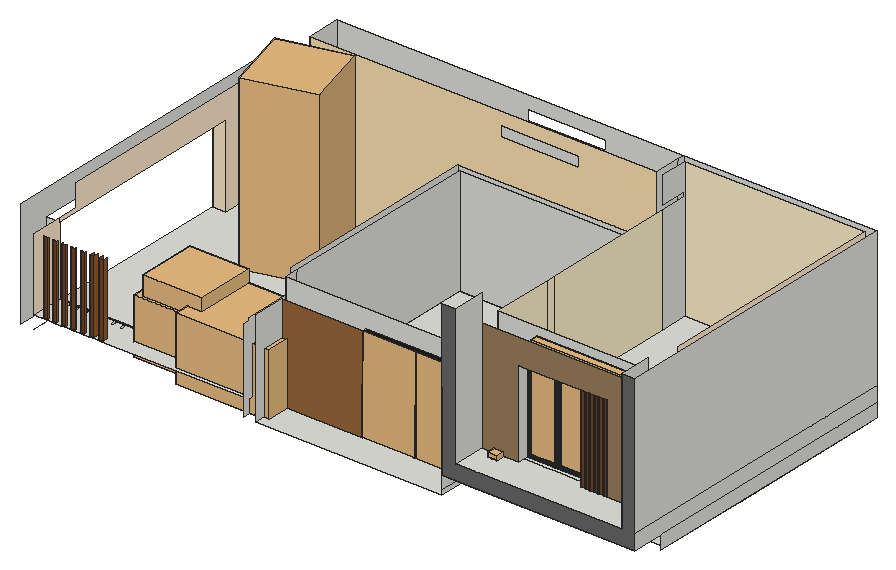
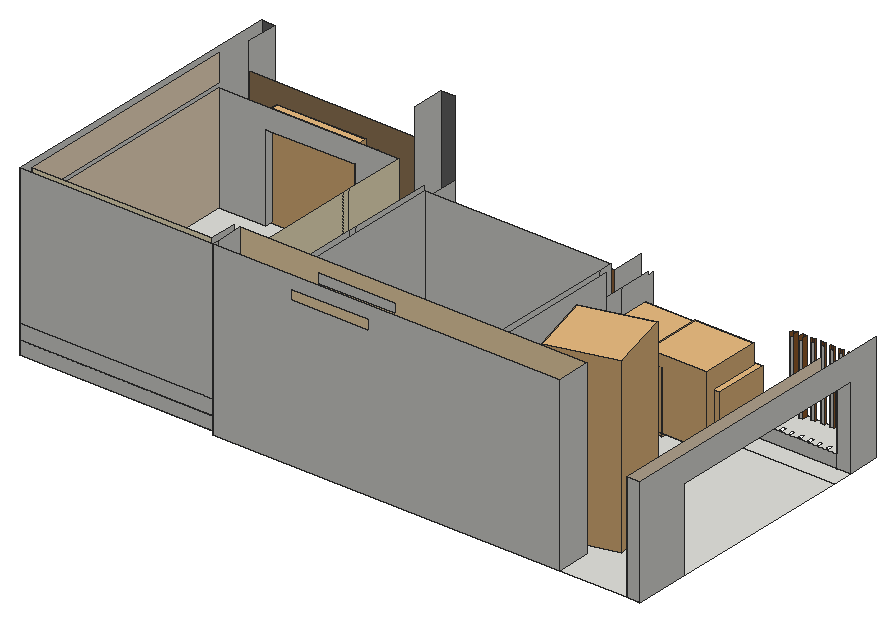
# SketchUp Ruby script. Lengths in inches.
U = 1.inch
M = Sketchup.active_model
def pt(a) = Geom::Point3d.new(a.map { |v| v * U })
def face(e, loops, mat)
  f = e.add_face(loops[0].map { |a| pt(a) })
  loops[1..].each { |l| e.add_face(l.map { |a| pt(a) }).erase! }
  f.material = f.back_material = mat if mat
  f
end
# faces: each face lists its corners as indices into pts; further lists are holes
def faces(e, pts, list, mat = nil) = list.each { |f| face(e, (f[0].is_a?(Array) ? f : [f]).map { |l| l.map { |i| pts[i] } }, mat) }
# xy, xz, yz: faces in a plane at the given z, y or x. An outline is a flat list of corners, or four numbers for a rectangle; further outlines are holes
def ring(l) = l.size == 4 ? [[l[0], l[1]], [l[2], l[1]], [l[2], l[3]], [l[0], l[3]]] : l.each_slice(2).to_a
def flat(e, list, mat, &to3) = list.each { |f| face(e, (f[0].is_a?(Array) ? f : [f]).map { |l| ring(l).map { |u, v| to3.(u, v) } }, mat) }
def xy(e, z, list, mat = nil) = flat(e, list, mat) { |x, y| [x, y, z] }
def xz(e, y, list, mat = nil) = flat(e, list, mat) { |x, z| [x, y, z] }
def yz(e, x, list, mat = nil) = flat(e, list, mat) { |y, z| [x, y, z] }
def lines(e, pts, list) = list.each { |a, b| e.add_line(pt(pts[a]), pt(pts[b])) }
# prism: a flat outline (further loops are holes) pulled along v
def prism(e, loops, v, mat = nil)
  f = face(e, loops, mat); d = Geom::Vector3d.new(v.map { |x| x * U })
  f.pushpull(f.normal.samedirection?(d) ? d.length : -d.length)
end
def box(e, o, s, mat = nil) = prism(e, [[o, [o[0] + s[0], o[1], o[2]], [o[0] + s[0], o[1] + s[1], o[2]], [o[0], o[1] + s[1], o[2]]]], [0, 0, s[2]], mat)
def at(x, y, z, deg = 0) = Geom::Transformation.translation(pt([x, y, z])) * Geom::Transformation.rotation(ORIGIN, Z_AXIS, deg.degrees)
def axes(o, x, y, z) = Geom::Transformation.new([*x, 0, *y, 0, *z, 0, *pt(o).to_a, 1])
def part(name) = M.definitions.add(name)
# library, detail: a bought-in or finely detailed component or shape, given as its bounding box
def library(name, o, s) = part(name).tap { |d| box(d.entities, o, s) }
def detail(e, o, s) = box(e.add_group.entities, o, s)
def put(e, d, t, mat = nil) = e.add_instance(d, t).tap { |i| i.material = mat if mat }
def group(e, t, mat = nil) = e.add_group.tap { |g| g.transformation = t; g.material = mat if mat }.entities
root = M.entities
M.materials.add("Wine2").color = [0, 0, 0]
M.materials["Wine2"].alpha = 0
M.materials.add("[0029_BlanchedAlmond]").color = [255, 235, 205]
M.materials.add("[0032_Moccasin]").color = [255, 228, 181]
M.materials.add("[0130_Gainsboro]").color = [39, 45, 50]
M.materials.add("[0134_DimGray]").color = [105, 105, 105]
M.materials.add("[Color D01]").color = [255, 242, 204]
M.materials.add("[Color M08]").color = [30, 30, 30]
M.materials.add("[Groundcover Sand Smooth]").color = [158, 128, 93]
M.materials.add("[Wood Floor Dark]").color = [153, 94, 42]
M.materials.add("[Wood Floor]").color = [155, 105, 61]
M.materials.add("[Wood Veneer 01]").color = [120, 70, 37]
c1 = library("Sem+nome (1)",[20.77,3.52,-2.22],[96.42,122.82,82.56])
c2 = library("Pot+Plant",[-20.81,-17.08,-0.03],[39.86,39.43,41.33])
c3 = library("staircases+paint",[157.6875,-222.19,0],[58.28,58.28,145.51])
c4 = library("1",[3.97,34.78,0],[101.43,33.99,0.79])
c5 = library("Floor plant",[-5.56,-16.3125,0.81],[76.88,76.71,92.33])
c6 = library("A$C06767DEF\#1",[-8.3,1.21,0],[7.09,7.09,5.51])
c7 = library("oeillet+feston+nino+blanc",[0,-1.53,0],[95.37,7.9,110.56])
c8 = part("Framed panel")
xy(c8.entities,0,[[0,-0.98,43.07,0],[0,0,43.07,1.4]],"[0130_Gainsboro]")
xy(c8.entities,0.3,[[0.3,-1.43,42.77,-0.98]],"[0130_Gainsboro]")
xy(c8.entities,2.95,[[2.95,-1.43,40.12,-0.63],[2.95,-0.63,40.12,0],[2.95,0,40.12,0.64],[2.95,0.64,40.12,1.4]],"[0130_Gainsboro]")
xy(c8.entities,3.54,[[3.54,-0.63,39.53,0],[3.54,0,39.53,0.64]],"[0130_Gainsboro]")
xy(c8.entities,111.8125,[[3.54,-0.63,39.53,0],[3.54,0,39.53,0.64]],"[0130_Gainsboro]")
xy(c8.entities,112.4,[[2.95,-1.43,40.12,-0.63],[2.95,-0.63,40.12,0],[2.95,0,40.12,0.64],[2.95,0.64,40.12,1.4]],"[0130_Gainsboro]")
xy(c8.entities,115.05,[[0.3,-1.43,42.77,-0.98]],"[0130_Gainsboro]")
xy(c8.entities,115.35,[[0,-0.98,43.07,0],[0,0,43.07,1.4]],"[0130_Gainsboro]")
xz(c8.entities,-1.43,[[[0.3,0.3,42.77,115.05],[2.95,2.95,40.12,112.4]]],"[0130_Gainsboro]")
xz(c8.entities,-0.98,[[[0,0,43.07,115.35],[0.3,0.3,42.77,115.05]]],"[0130_Gainsboro]")
xz(c8.entities,-0.63,[[[2.95,2.95,40.12,112.4],[3.54,3.54,39.53,111.8125]]],"[0130_Gainsboro]")
xz(c8.entities,0,[[3.54,3.54,39.53,111.8125]],"Wine2")
xz(c8.entities,0,[[[0,0,43.07,115.35],[2.95,2.95,40.12,112.4]],[[2.95,2.95,40.12,112.4],[3.54,3.54,39.53,111.8125]]],"[0130_Gainsboro]")
xz(c8.entities,0.64,[[[2.95,2.95,40.12,112.4],[3.54,3.54,39.53,111.8125]]],"[0130_Gainsboro]")
xz(c8.entities,1.4,[[[0,0,43.07,115.35],[2.95,2.95,40.12,112.4]]],"[0130_Gainsboro]")
yz(c8.entities,0,[[-0.98,0,0,115.35],[0,0,1.4,115.35]],"[0130_Gainsboro]")
yz(c8.entities,0.3,[[-1.43,0.3,-0.98,115.05]],"[0130_Gainsboro]")
yz(c8.entities,2.95,[[-1.43,2.95,-0.63,112.4],[-0.63,2.95,0,112.4],[0,2.95,0.64,112.4],[0.64,2.95,1.4,112.4]],"[0130_Gainsboro]")
yz(c8.entities,3.54,[[-0.63,3.54,0,111.8125],[0,3.54,0.64,111.8125]],"[0130_Gainsboro]")
yz(c8.entities,39.53,[[-0.63,3.54,0,111.8125],[0,3.54,0.64,111.8125]],"[0130_Gainsboro]")
yz(c8.entities,40.12,[[-1.43,2.95,-0.63,112.4],[-0.63,2.95,0,112.4],[0,2.95,0.64,112.4],[0.64,2.95,1.4,112.4]],"[0130_Gainsboro]")
yz(c8.entities,42.77,[[-1.43,0.3,-0.98,115.05]],"[0130_Gainsboro]")
yz(c8.entities,43.07,[[-0.98,0,0,115.35],[0,0,1.4,115.35]],"[0130_Gainsboro]")
c9 = part("Framed panel assembly")
put(c9.entities,c8,axes([90.57,1.43,0],[1.05148,0,0],[0,1,0],[0,0,1]))
put(c9.entities,c8,axes([0,1.43,0],[1.05148,0,0],[0,1,0],[0,0,1]))
put(c9.entities,c8,axes([45.29,1.43,0],[1.05148,0,0],[0,1,0],[0,0,1]))
xy(root,146.375,[[416.52,389.67,660.05,389.67,660.05,437.41,522.24,437.41,522.24,431.86,416.52,431.86],[522.24,437.41,660.05,440.22],[101.6875,440.22,400.76,466.49],[[400.76,440.22,660.05,739.86],[408.8,448.26,652.01,731.82]],[408.8,448.26,652.01,731.82],
  [101.6875,466.49,400.76,466.49,400.76,739.86,207.07,739.86,207.07,784.05,118.89,784.05,118.89,712.1,101.6875,712.1],[101.6875,712.1,118.89,784.05],[207.07,739.86,660.05,784.05]])
xy(root,151.4375,[[660.05,440.22,666.61,551.1875],[666.61,440.22,904.08,551.1875],[904.08,440.22,912.4375,551.1875],[660.05,551.1875,666.61,562.07],[666.61,551.1875,904.08,562.07],
  [904.08,551.1875,912.4375,562.07],[660.05,562.07,904.08,775.6875],[904.08,562.07,912.4375,775.6875],[660.05,775.6875,912.4375,784.05]])
xy(root,163.5625,[[[118.89,397.92,130.43,397.92,130.43,401.21,135.74,401.21,135.74,397.92,142.61,397.92,142.61,401.21,147.93,401.21,147.93,397.92,154.8,397.92,154.8,401.21,160.11,401.21,160.11,397.92,166.99,397.92,166.99,401.21,172.3,401.21,172.3,397.92,179.18,397.92,179.18,401.21,184.49,401.21,184.49,397.92,191.36,397.92,191.36,405.64,196.68,405.64,196.68,397.92,203.55,397.92,203.55,405.01,208.86,405.01,208.86,397.92,400.76,397.92,400.76,440.22,118.89,440.22],[179.18,431.86,184.49,438.86],[203.55,431.86,208.86,438.86],[191.36,431.86,196.68,438.86],[130.43,431.86,135.74,438.86],[166.99,431.86,172.3,438.86],[142.61,431.86,147.93,438.86],[154.8,431.86,160.11,438.86]],[130.43,397.92,135.74,399.67],[142.61,397.92,147.93,399.67],[154.8,397.92,160.11,399.67],[166.99,397.92,172.3,399.67],
  [179.18,397.92,184.49,399.67],[191.36,397.92,196.68,399.67],[203.55,397.92,208.86,399.67]])
xy(root,169.25,[[660.05,389.67,660.05,784.05,912.4375,784.05,912.4375,431.86,798.1,431.86,798.1,432.24,795.91,432.24,795.91,431.86,720.28,431.86,720.28,432.24,713.72,432.24,713.72,433.11,711.84,433.11,711.84,432.24,705.28,432.24,705.28,433.11,703.41,433.11,703.41,432.17,696.84,432.17,696.84,433.11,694.97,433.11,694.97,432.17,688.41,432.17,688.41,433.11,686.53,433.11,686.53,432.17,679.97,432.17,679.97,433.11,678.11,433.11,678.11,389.67]])
xy(root,169.25,[[678.11,389.67,678.11,433.11,679.97,433.11,679.97,432.17,686.53,432.17,686.53,433.11,688.41,433.11,688.41,432.17,694.97,432.17,694.97,433.11,696.84,433.11,696.84,432.17,703.41,432.17,703.41,433.11,705.28,433.11,705.28,432.24,711.84,432.24,711.84,433.11,713.72,433.11,713.72,432.24,720.28,432.24,720.28,431.86,795.91,431.86,795.91,432.24,798.1,432.24,798.1,431.86,912.4375,431.86,912.4375,389.67]],"[Wood Floor Dark]")
xy(root,185.875,[[699.62,420.82,701.17,421.02,702.625,421.62,703.87,422.56,704.83,423.8,705.43,425.25,705.64,426.8,705.45,428.35,704.85,429.8,703.9,431.05,702.86,431.86,696.44,431.86,695.42,431.08,694.46,429.85,693.86,428.4,693.64,426.85,693.84,425.29,694.4375,423.85,695.39,422.6,696.625,421.64,698.07,421.03],[875.48,421.71,877.03,421.92,878.48,422.52,879.72,423.47,880.67,424.71,881.27,426.16,881.48,427.71,881.27,429.27,880.67,430.71,879.79,431.86,871.16,431.86,870.28,430.71,869.68,429.27,869.48,427.71,869.68,426.16,870.28,424.71,871.23,423.47,872.48,422.52,873.92,421.92]])
xy(root,188.9375,[[[678.11,389.67,895.55,389.67,895.55,431.86,879.79,431.86,880.67,430.71,881.27,429.27,881.48,427.71,881.27,426.16,880.67,424.71,879.72,423.47,878.48,422.52,877.03,421.92,875.48,421.71,873.92,421.92,872.48,422.52,871.23,423.47,870.28,424.71,869.68,426.16,869.48,427.71,869.68,429.27,870.28,430.71,871.16,431.86,837.78,431.86,837.78,434.99,842.22,434.99,842.22,440.41,726.09,440.41,726.09,431.86,702.86,431.86,703.9,431.05,704.85,429.8,705.45,428.35,705.64,426.8,705.43,425.25,704.83,423.8,703.87,422.56,702.625,421.62,701.17,421.02,699.62,420.82,698.07,421.03,696.625,421.64,695.39,422.6,694.4375,423.85,693.84,425.29,693.64,426.85,693.86,428.4,694.46,429.85,695.42,431.08,696.44,431.86,678.11,431.86],[807.9,431.86,812.34,434.99],[813.9,431.86,818.34,434.99],[819.9,431.86,824.34,434.99],[825.9,431.86,830.34,434.99],[831.78,431.86,836.22,434.99]],[696.44,431.86,702.86,431.86,702.67,432.01,701.22,432.61,699.67,432.82,698.12,432.625,696.67,432.03],[871.16,431.86,879.79,431.86,879.72,431.96,878.48,432.91,877.03,433.51,875.48,433.71,873.92,433.51,872.48,432.91,871.23,431.96],[726.09,440.41,842.22,440.41,842.22,469.66,903.88,469.66,903.88,775.49,668.6,775.49,668.6,469.66,726.09,469.66]])
xz(root,389.67,[[660.05,169.25,912.4375,169.25,912.4375,370.4375,895.55,370.4375,895.55,188.9375,678.11,188.9375,678.11,370.4375,660.05,370.4375]],"[0134_DimGray]")
xz(root,399.67,[[130.43,163.5625,135.74,258.66],[142.61,163.5625,147.93,258.66],[154.8,163.5625,160.11,258.66],[166.99,163.5625,172.3,258.66],[179.18,163.5625,184.49,258.66],
  [191.36,163.5625,196.68,258.66],[203.55,163.5625,208.86,258.66]],"[Wood Veneer 01]")
xz(root,401.21,[[130.43,163.5625,135.74,254.91],[142.61,163.5625,147.93,254.91],[154.8,163.5625,160.11,254.91],[166.99,163.5625,172.3,254.91],[179.18,163.5625,184.49,254.91]])
xz(root,405.01,[[203.55,163.5625,208.86,254.91]])
xz(root,405.64,[[191.36,163.5625,196.68,254.91]])
xz(root,431.86,[[696.44,185.875,702.86,188.9375],[871.16,185.875,879.79,188.9375]])
xz(root,431.86,[[678.11,188.9375,726.09,188.9375,726.09,302.375,842.22,302.375,842.22,188.9375,895.55,188.9375,895.55,335.3125,678.11,335.3125]],"[Groundcover Sand Smooth]")
xz(root,431.86,[[416.52,146.375,522.24,271.24]],"[Wood Floor]")
xz(root,431.86,[[807.9,188.9375,812.34,302.375],[813.9,188.9375,818.34,302.375],[819.9,188.9375,824.34,302.375],[825.9,188.9375,830.34,302.375],[831.78,188.9375,836.22,302.375],
  [837.78,188.9375,842.22,302.375]],"[Wood Veneer 01]")
xz(root,434.99,[[807.9,188.9375,812.34,302.375],[813.9,188.9375,818.34,302.375],[819.9,188.9375,824.34,302.375],[825.9,188.9375,830.34,302.375],[831.78,188.9375,836.22,302.375],
  [837.78,188.9375,842.22,302.375]])
xz(root,437.41,[[522.24,146.375,660.05,271.24]],"[Color M08]")
xz(root,440.22,[[101.6875,146.375,118.89,253.6875],[118.89,146.375,400.76,163.5625]])
xz(root,448.26,[[408.8,146.375,652.01,287.5625]])
xz(root,469.66,[[668.6,188.9375,668.6,329.3125,903.88,329.3125,903.88,188.9375,842.22,188.9375,842.22,302.375,726.09,302.375,726.09,188.9375]])
xz(root,712.1,[[101.6875,146.375,118.89,253.6875]],"[0029_BlanchedAlmond]")
xz(root,731.82,[[408.8,146.375,652.01,287.5625]])
xz(root,739.86,[[400.76,146.375,660.05,287.5625]])
xz(root,739.86,[[[207.07,146.375,400.76,146.375,400.76,287.5625,660.05,287.5625,660.05,370.4375,207.07,370.4375],[456.09,340.08,558.27,353.76]]],"[0032_Moccasin]")
xz(root,775.49,[[668.6,188.9375,903.88,370.4375]],"[Color D01]")
xz(root,784.05,[[101.6875,146.375,118.89,287.5625],[[207.07,146.375,660.05,370.4375],[456.09,340.08,558.27,353.76]],[660.05,151.4375,912.4375,169.25],[660.05,169.25,912.4375,188.9375],[660.05,188.9375,912.4375,370.4375]])
yz(root,101.6875,[[397.92,146.375,397.92,287.5625,784.05,287.5625,784.05,146.375,712.1,146.375,712.1,253.6875,440.22,253.6875,440.22,146.375]])
yz(root,118.89,[[712.1,146.375,784.05,146.375,784.05,287.5625,466.49,287.5625,466.49,258.66,440.22,258.66,440.22,253.6875,712.1,253.6875],[397.92,163.5625,440.22,258.66]],"[0029_BlanchedAlmond]")
yz(root,130.43,[[399.67,163.5625,401.21,258.66]],"[Wood Floor Dark]")
yz(root,135.74,[[399.67,163.5625,401.21,258.66]],"[Wood Floor Dark]")
yz(root,142.61,[[399.67,163.5625,401.21,258.66]],"[Wood Floor Dark]")
yz(root,147.93,[[399.67,163.5625,401.21,258.66]],"[Wood Floor Dark]")
yz(root,154.8,[[399.67,163.5625,401.21,258.66]],"[Wood Floor Dark]")
yz(root,160.11,[[399.67,163.5625,401.21,258.66]],"[Wood Floor Dark]")
yz(root,166.99,[[399.67,163.5625,401.21,258.66]],"[Wood Floor Dark]")
yz(root,172.3,[[399.67,163.5625,401.21,258.66]],"[Wood Floor Dark]")
yz(root,179.18,[[399.67,163.5625,401.21,258.66]],"[Wood Floor Dark]")
yz(root,184.49,[[399.67,163.5625,401.21,258.66]],"[Wood Floor Dark]")
yz(root,191.36,[[399.67,163.5625,405.64,258.66]],"[Wood Floor Dark]")
yz(root,196.68,[[399.67,163.5625,405.64,258.66]],"[Wood Floor Dark]")
yz(root,203.55,[[399.67,163.5625,399.67,258.66,404.92,258.66,404.92,254.91,405.01,254.91,405.01,163.5625]],"[Wood Floor Dark]")
yz(root,207.07,[[739.86,146.375,784.05,370.4375]])
yz(root,208.86,[[399.67,163.5625,405.01,163.5625,405.01,254.91,404.92,254.91,404.92,258.66,399.67,258.66]],"[Wood Floor Dark]")
yz(root,400.76,[[389.67,146.375,389.67,254.91,397.92,254.91,397.92,258.66,440.22,258.66,440.22,163.5625,397.92,163.5625,397.92,146.375],[440.22,146.375,466.49,258.66],[466.49,146.375,739.86,287.5625]])
yz(root,408.8,[[448.26,146.375,466.49,287.5625],[466.49,146.375,731.82,287.5625]])
yz(root,416.52,[[389.67,146.375,431.86,271.24]])
yz(root,522.24,[[431.86,146.375,437.41,271.24]])
yz(root,652.01,[[448.26,146.375,731.82,287.5625]])
yz(root,660.05,[[389.67,146.375,437.41,151.4375],[437.41,146.375,551.1875,151.4375],[551.1875,146.375,562.07,151.4375],[562.07,146.375,739.86,151.4375],[739.86,146.375,775.6875,151.4375],
  [775.6875,146.375,784.05,151.4375],[389.67,151.4375,437.41,169.25],[437.41,151.4375,551.1875,169.25],[551.1875,151.4375,562.07,169.25],[562.07,151.4375,739.86,169.25],
  [739.86,151.4375,775.6875,169.25],[775.6875,151.4375,784.05,169.25],[389.67,169.25,437.41,188.9375],[437.41,169.25,551.1875,188.9375],[551.1875,169.25,562.07,188.9375],
  [562.07,169.25,739.86,188.9375],[739.86,169.25,775.6875,188.9375],[775.6875,169.25,784.05,188.9375],[389.67,188.9375,437.41,271.24],[437.41,188.9375,437.41,271.24,440.22,271.24,440.22,287.5625,551.1875,287.5625,551.1875,188.9375],
  [551.1875,188.9375,562.07,287.5625],[562.07,188.9375,739.86,287.5625],[739.86,188.9375,775.6875,370.4375],[775.6875,188.9375,784.05,370.4375]])
yz(root,668.6,[[739.86,188.9375,775.49,188.9375,775.49,370.4375,739.86,370.4375,739.86,335.3125,774.73,335.3125,774.73,329.3125,739.86,329.3125]])
yz(root,668.6,[[469.66,188.9375,551.1875,329.3125],[551.1875,188.9375,562.07,329.3125],[562.07,188.9375,739.86,329.3125]],"[Color D01]")
yz(root,678.11,[[389.67,188.9375,431.86,370.4375]])
yz(root,726.09,[[431.86,188.9375,469.66,302.375]])
yz(root,807.9,[[431.86,188.9375,434.99,302.375]])
yz(root,812.34,[[431.86,188.9375,434.99,302.375]])
yz(root,813.9,[[431.86,188.9375,434.99,302.375]])
yz(root,818.34,[[431.86,188.9375,434.99,302.375]])
yz(root,819.9,[[431.86,188.9375,434.99,302.375]])
yz(root,824.34,[[431.86,188.9375,434.99,302.375]])
yz(root,825.9,[[431.86,188.9375,434.99,302.375]])
yz(root,830.34,[[431.86,188.9375,434.99,302.375]])
yz(root,831.78,[[431.86,188.9375,434.99,302.375]])
yz(root,836.22,[[431.86,188.9375,434.99,302.375]])
yz(root,837.78,[[431.86,188.9375,434.99,302.375]])
yz(root,842.22,[[431.86,188.9375,434.99,302.375],[434.99,188.9375,469.66,302.375]])
yz(root,895.55,[[389.67,188.9375,431.86,370.4375]])
yz(root,903.88,[[469.66,188.9375,469.66,329.3125,774.73,329.3125,774.73,335.3125,469.66,335.3125,469.66,370.4375,775.49,370.4375,775.49,188.9375]],"[0029_BlanchedAlmond]")
yz(root,912.4375,[[431.86,151.4375,784.05,169.25],[389.67,169.25,784.05,188.9375],[389.67,188.9375,784.05,370.4375]])
p = [[698.07,421.03,188.9375],[699.62,420.82,188.9375],[699.62,420.82,185.875],[698.07,421.03,185.875],[701.17,421.02,188.9375],[701.17,421.02,185.875],
  [696.625,421.64,188.9375],[696.625,421.64,185.875],[702.625,421.62,188.9375],[702.625,421.62,185.875],[695.39,422.6,188.9375],[695.39,422.6,185.875],
  [703.87,422.56,188.9375],[703.87,422.56,185.875],[873.92,421.92,188.9375],[875.48,421.71,188.9375],[875.48,421.71,185.875],[873.92,421.92,185.875],
  [877.03,421.92,188.9375],[877.03,421.92,185.875],[872.48,422.52,188.9375],[872.48,422.52,185.875],[878.48,422.52,188.9375],[878.48,422.52,185.875],
  [871.23,423.47,188.9375],[871.23,423.47,185.875],[879.72,423.47,188.9375],[879.72,423.47,185.875],[694.4375,423.85,188.9375],[694.4375,423.85,185.875],
  [704.83,423.8,188.9375],[704.83,423.8,185.875],[870.28,424.71,188.9375],[870.28,424.71,185.875],[880.67,424.71,188.9375],[880.67,424.71,185.875],
  [693.84,425.29,188.9375],[693.84,425.29,185.875],[705.43,425.25,188.9375],[705.43,425.25,185.875],[869.68,426.16,188.9375],[869.68,426.16,185.875],
  [881.27,426.16,188.9375],[881.27,426.16,185.875],[705.64,426.8,188.9375],[705.64,426.8,185.875],[693.64,426.85,188.9375],[693.64,426.85,185.875],
  [869.48,427.71,188.9375],[869.48,427.71,185.875],[881.48,427.71,188.9375],[881.48,427.71,185.875],[693.86,428.4,188.9375],[693.86,428.4,185.875],
  [705.45,428.35,188.9375],[705.45,428.35,185.875],[869.68,429.27,188.9375],[869.68,429.27,185.875],[881.27,429.27,188.9375],[881.27,429.27,185.875],
  [694.46,429.85,188.9375],[694.46,429.85,185.875],[704.85,429.8,188.9375],[704.85,429.8,185.875],[870.28,430.71,188.9375],[870.28,430.71,185.875],
  [880.67,430.71,188.9375],[880.67,430.71,185.875],[695.42,431.08,188.9375],[695.42,431.08,185.875],[703.9,431.05,188.9375],[703.9,431.05,185.875],
  [871.16,431.86,188.9375],[871.16,431.86,185.875],[879.79,431.86,188.9375],[879.79,431.86,185.875],[702.86,431.86,188.9375],[702.86,431.86,185.875],
  [696.44,431.86,188.9375],[696.44,431.86,185.875],[118.89,440.22,146.375],[118.89,397.92,146.375],[1156.02,89.3,146.44],[1155.6,88.88,146.44],
  [1156.02,88.88,146.44]]
faces(root,p,[[0,1,2,3],[1,4,5,2],[6,0,3,7],[4,8,9,5],[10,6,7,11],[8,12,13,9],[14,15,16,17],[15,18,19,16],
  [20,14,17,21],[18,22,23,19],[24,20,21,25],[22,26,27,23],[28,10,11,29],[12,30,31,13],[32,24,25,33],[26,34,35,27],
  [36,28,29,37],[30,38,39,31],[40,32,33,41],[34,42,43,35],[38,44,45,39],[46,36,37,47],[48,40,41,49],[42,50,51,43],
  [52,46,47,53],[44,54,55,45],[56,48,49,57],[50,58,59,51],[60,52,53,61],[54,62,63,55],[64,56,57,65],[58,66,67,59],
  [68,60,61,69],[62,70,71,63],[72,64,65,73],[66,74,75,67],[70,76,77,71],[78,68,69,79]])
lines(root,p,[[80,81],[82,83],[83,84],[84,82]])
put(root,c1,at(296.83,520.26,146.3125,-90))
put(root,c2,axes([269.95,449.73,145.03],[1.76,0,0],[0,1.76,0],[0,0,1.76]))
put(root,c3,axes([-118.9,895.33,146.375],[1.48753,0.39858,0],[-0.39858,1.48753,0],[0,0,1.54]),"[0032_Moccasin]")
put(root,c4,axes([664.46,431.55,142.65],[0,0.01041,1.21996],[-2.0679,0,0],[0,-1.21996,0.01041]))
put(root,c4,axes([730.71,431.1,142.65],[0,0.01041,1.21996],[-2.013,0,0],[0,-1.21996,0.01041]))
put(root,c5,at(247.15,439.48,149.4))
put(root,c6,axes([867.46,420.13,194.45],[-1.72643,0,0],[0,1.41388,0],[0,0,-1.23]))
put(root,c6,axes([691.89,420.13,194.45],[-1.72643,0,0],[0,1.41388,0],[0,0,-1.23]))
put(root,c7,axes([726.09,453.64,188.9375],[1.22,0,0],[0,1.22,0],[0,0,1.22]))
put(root,c9,axes([726.73,446.27,188.9375],[0.85,0,0],[0,0.85,0],[0,0,0.98338]))
